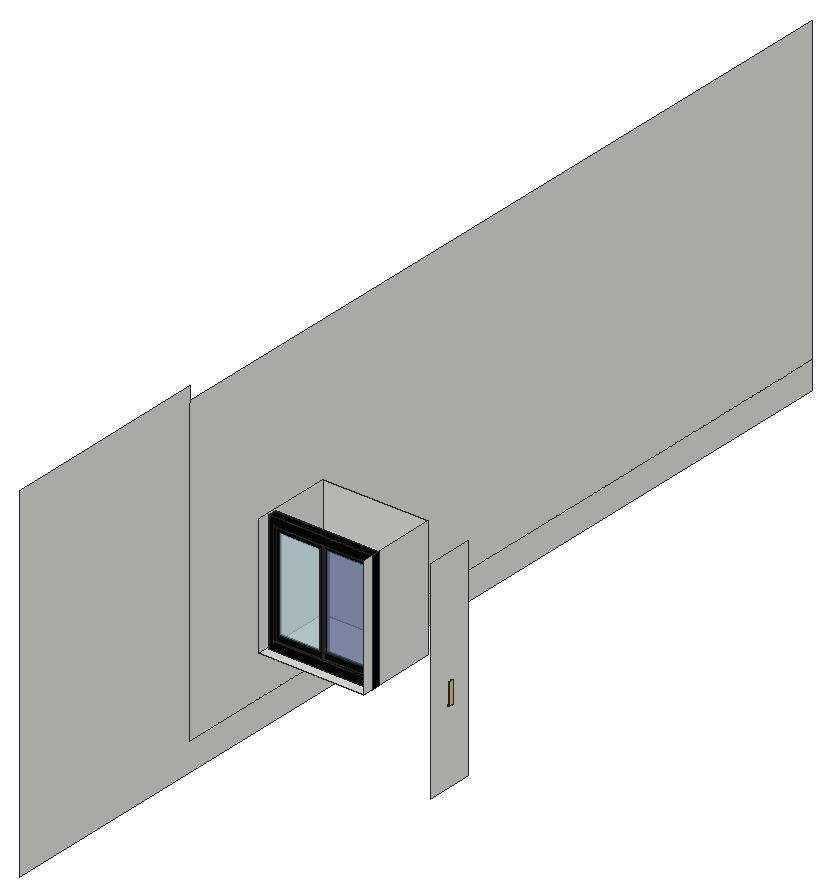
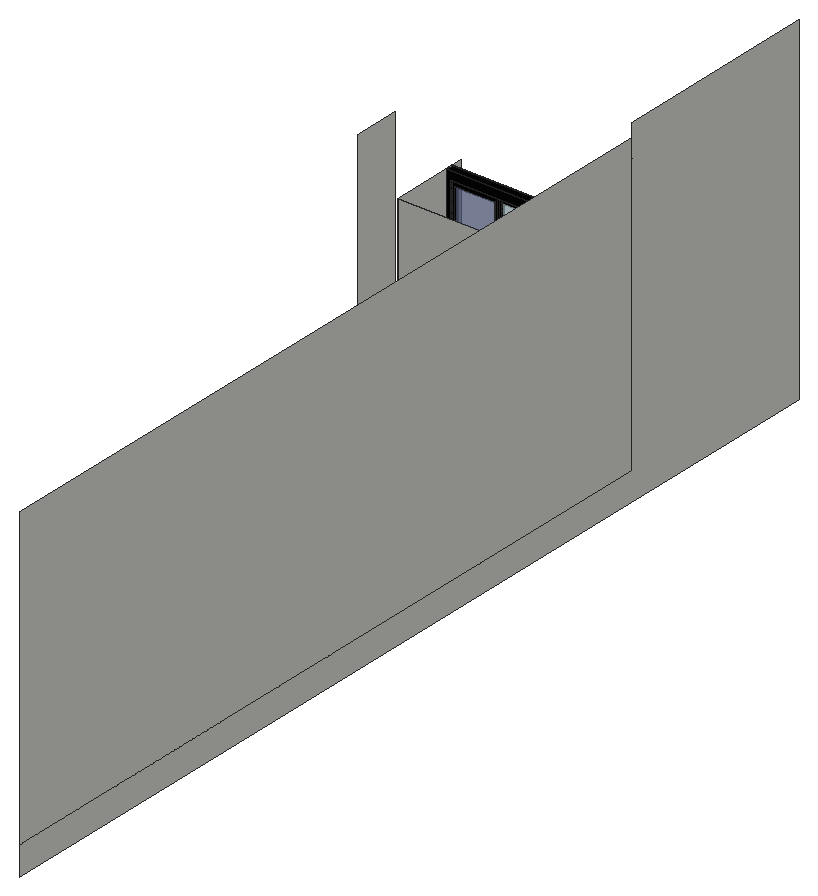
# SketchUp Ruby script. Lengths in inches.
U = 1.inch
M = Sketchup.active_model
def pt(a) = Geom::Point3d.new(a.map { |v| v * U })
def face(e, loops, mat)
  f = e.add_face(loops[0].map { |a| pt(a) })
  loops[1..].each { |l| e.add_face(l.map { |a| pt(a) }).erase! }
  f.material = f.back_material = mat if mat
  f
end
# faces: each face lists its corners as indices into pts; further lists are holes
def faces(e, pts, list, mat = nil) = list.each { |f| face(e, (f[0].is_a?(Array) ? f : [f]).map { |l| l.map { |i| pts[i] } }, mat) }
# xy, xz, yz: faces in a plane at the given z, y or x. An outline is a flat list of corners, or four numbers for a rectangle; further outlines are holes
def ring(l) = l.size == 4 ? [[l[0], l[1]], [l[2], l[1]], [l[2], l[3]], [l[0], l[3]]] : l.each_slice(2).to_a
def flat(e, list, mat, &to3) = list.each { |f| face(e, (f[0].is_a?(Array) ? f : [f]).map { |l| ring(l).map { |u, v| to3.(u, v) } }, mat) }
def xy(e, z, list, mat = nil) = flat(e, list, mat) { |x, y| [x, y, z] }
def xz(e, y, list, mat = nil) = flat(e, list, mat) { |x, z| [x, y, z] }
def yz(e, x, list, mat = nil) = flat(e, list, mat) { |y, z| [x, y, z] }
def lines(e, pts, list) = list.each { |a, b| e.add_line(pt(pts[a]), pt(pts[b])) }
# prism: a flat outline (further loops are holes) pulled along v
def prism(e, loops, v, mat = nil)
  f = face(e, loops, mat); d = Geom::Vector3d.new(v.map { |x| x * U })
  f.pushpull(f.normal.samedirection?(d) ? d.length : -d.length)
end
def box(e, o, s, mat = nil) = prism(e, [[o, [o[0] + s[0], o[1], o[2]], [o[0] + s[0], o[1] + s[1], o[2]], [o[0], o[1] + s[1], o[2]]]], [0, 0, s[2]], mat)
def at(x, y, z, deg = 0) = Geom::Transformation.translation(pt([x, y, z])) * Geom::Transformation.rotation(ORIGIN, Z_AXIS, deg.degrees)
def axes(o, x, y, z) = Geom::Transformation.new([*x, 0, *y, 0, *z, 0, *pt(o).to_a, 1])
def part(name) = M.definitions.add(name)
# library, detail: a bought-in or finely detailed component or shape, given as its bounding box
def library(name, o, s) = part(name).tap { |d| box(d.entities, o, s) }
def detail(e, o, s) = box(e.add_group.entities, o, s)
def put(e, d, t, mat = nil) = e.add_instance(d, t).tap { |i| i.material = mat if mat }
def group(e, t, mat = nil) = e.add_group.tap { |g| g.transformation = t; g.material = mat if mat }.entities
root = M.entities
M.materials.add("Generic\#5").color = [7, 6, 6]
M.materials.add("Material \#1").color = [140, 140, 140]
M.materials.add("[Translucent_Glass_Safety]").color = [204, 235, 244]
M.materials["[Translucent_Glass_Safety]"].alpha = 0.5
M.materials.add("[Translucent_Glass_Sky_Reflection]").color = [125, 138, 183]
M.materials["[Translucent_Glass_Sky_Reflection]"].alpha = 0.52
c1 = part("Sliding window")
xy(c1.entities,0,[[0,0,4.33,55.51]])
xy(c1.entities,2.76,[[0,2.76,2,27.76],[3.15,2.76,4.33,27.76],[0,27.76,0.82,52.76],[0.82,27.76,2.36,52.76],[2.36,27.76,4.33,52.76]])
xy(c1.entities,4.72,[[2,4.72,2.4,26.38],[2.76,4.72,3.15,26.38],[0.82,29.13,1.22,50.79],[1.97,29.13,2.36,50.79]])
xy(c1.entities,36.61,[[2,4.72,2.4,26.38],[2.76,4.72,3.15,26.38],[0.82,29.13,1.22,50.79],[1.97,29.13,2.36,50.79]])
xy(c1.entities,38.58,[[0,2.76,2,27.76],[3.15,2.76,4.33,27.76],[0,27.76,0.82,52.76],[0.82,27.76,2.36,52.76],[2.36,27.76,4.33,52.76]])
xy(c1.entities,41.34,[[0,0,4.33,55.51]])
xz(c1.entities,0,[[0,0,4.33,41.34]])
xz(c1.entities,2.76,[[0,2.76,2,38.58],[3.15,2.76,4.33,38.58]])
xz(c1.entities,4.72,[[2,4.72,2.4,36.61],[2.76,4.72,3.15,36.61]])
xz(c1.entities,26.38,[[2,4.72,2.4,36.61],[2.76,4.72,3.15,36.61]])
xz(c1.entities,27.76,[[0.82,2.76,2,38.58],[2,2.76,2.36,38.58],[2.36,2.76,3.15,38.58]])
xz(c1.entities,29.13,[[0.82,4.72,1.22,36.61],[1.97,4.72,2.36,36.61]])
xz(c1.entities,50.79,[[0.82,4.72,1.22,36.61],[1.97,4.72,2.36,36.61]])
xz(c1.entities,52.76,[[0,2.76,0.82,38.58],[0.82,2.76,2.36,38.58],[2.36,2.76,4.33,38.58]])
xz(c1.entities,55.51,[[0,0,4.33,41.34]])
yz(c1.entities,0,[[[0,0,55.51,41.34],[2.76,2.76,52.76,38.58]]])
yz(c1.entities,0.82,[[[27.76,2.76,52.76,38.58],[29.13,4.72,50.79,36.61]]])
yz(c1.entities,1.22,[[29.13,4.72,50.79,36.61]],"[Translucent_Glass_Sky_Reflection]")
yz(c1.entities,1.97,[[29.13,4.72,50.79,36.61]],"[Translucent_Glass_Sky_Reflection]")
yz(c1.entities,2,[[[2.76,2.76,27.76,38.58],[4.72,4.72,26.38,36.61]]])
yz(c1.entities,2.36,[[[27.76,2.76,52.76,38.58],[29.13,4.72,50.79,36.61]]])
yz(c1.entities,2.4,[[4.72,4.72,26.38,36.61]],"[Translucent_Glass_Safety]")
yz(c1.entities,2.76,[[4.72,4.72,26.38,36.61]],"[Translucent_Glass_Safety]")
yz(c1.entities,3.15,[[[2.76,2.76,27.76,38.58],[4.72,4.72,26.38,36.61]]])
yz(c1.entities,4.33,[[[0,0,55.51,41.34],[2.76,2.76,52.76,38.58]]])
c2 = library("3DGeom~4_Defintion",[-18.02,-499.97,-221.16],[36.04,1000,262.12])
c3 = part("3DGeom~5_Defintion")
xy(c3.entities,-225.24,[[-0.79,-499.98,-2.33,-499.64,7.45,-496.14],[-0.79,-499.98,7.45,-496.14,1.58,-499.88],[1.58,-499.88,7.45,-496.14,3.84,-499.16],[-2.33,-499.64,7.4,-485.75,7.45,-496.14],[3.84,-499.16,7.45,-496.14,5.85,-497.89],
  [7.45,-496.14,7.4,-485.75,8.24,-487.08],[7.45,-496.14,8.24,-487.08,8.96,-489.34],[7.45,-496.14,8.96,-489.34,9.0625,-491.71],[7.45,-496.14,9.0625,-491.71,8.55,-494.03],[-7.4,-496.08,-8.24,-494.76,2.32,-482.2],
  [-8.24,-494.76,-8.96,-492.5,2.32,-482.2],[-8.96,-492.5,-9.0625,-490.125,2.32,-482.2],[-9.0625,-490.125,-8.55,-487.81,2.32,-482.2],[-8.55,-487.81,-7.45,-485.7,2.32,-482.2],[-7.45,-485.7,-5.85,-483.95,2.32,-482.2],
  [-5.85,-483.95,-3.84,-482.68,2.32,-482.2],[-3.84,-482.68,-1.58,-481.96,2.32,-482.2],[2.32,-482.2,-1.58,-481.96,0.79,-481.86],[0,481.82,-2.35,482.13,-6.92,496.71],[0,481.82,-6.92,496.71,1.55,482.04],
  [-2.35,482.13,-4.55,483.04,-6.92,496.71],[-4.55,483.04,-6.43,484.49,-6.92,496.71],[-6.43,484.49,-7.88,486.37,-6.92,496.71],[6.92,485.12,-1.55,499.8125,7.88,495.47],[6.92,485.12,7.88,495.47,7.88,486.37],
  [-7.88,486.37,-8.79,488.57,-6.92,496.71],[7.88,486.37,7.88,495.47,8.79,488.57],[-8.79,488.57,-9.1,490.92,-6.92,496.71],[8.79,488.57,7.88,495.47,9.1,490.92],[-9.1,490.92,-8.79,493.28,-6.92,496.71],
  [9.1,490.92,7.88,495.47,8.79,493.28],[-8.79,493.28,-7.88,495.47,-6.92,496.71],[7.88,495.47,-1.55,499.8125,0,500.02],[7.88,495.47,0,500.02,2.35,499.71],[7.88,495.47,2.35,499.71,4.55,498.8],
  [7.88,495.47,4.55,498.8,6.43,497.35]],"Material \#1")
xy(c3.entities,-221.57,[[-2.33,-499.64,-5.22,-498.37,7.4,-485.75],[-5.22,-498.37,-7.4,-496.08,5.22,-483.47],[-5.22,-498.37,5.22,-483.47,7.4,-485.75],[-7.4,-496.08,2.32,-482.2,5.22,-483.47],[1.55,482.04,-6.92,496.71,-4.55,498.8],
  [1.55,482.04,-4.55,498.8,4.55,483.04],[4.55,483.04,-4.55,498.8,-1.55,499.8125],[4.55,483.04,-1.55,499.8125,6.92,485.12]],"Material \#1")
xy(c3.entities,38.05,[[-2.33,-499.64,7.4,-485.75,-5.22,-498.37],[-5.22,-498.37,5.22,-483.47,-7.4,-496.08],[-5.22,-498.37,7.4,-485.75,5.22,-483.47],[-7.4,-496.08,5.22,-483.47,2.32,-482.2],[1.55,482.04,-4.55,498.8,-6.92,496.71],
  [1.55,482.04,4.55,483.04,-4.55,498.8],[4.55,483.04,-1.55,499.8125,-4.55,498.8],[4.55,483.04,6.92,485.12,-1.55,499.8125]],"Material \#1")
xy(c3.entities,41.72,[[-0.79,-499.98,7.45,-496.14,-2.33,-499.64],[-0.79,-499.98,1.58,-499.88,7.45,-496.14],[1.58,-499.88,3.84,-499.16,7.45,-496.14],[-2.33,-499.64,7.45,-496.14,7.4,-485.75],[3.84,-499.16,5.85,-497.89,7.45,-496.14],
  [7.45,-496.14,8.24,-487.08,7.4,-485.75],[7.45,-496.14,8.55,-494.03,9.0625,-491.71],[7.45,-496.14,8.96,-489.34,8.24,-487.08],[7.45,-496.14,9.0625,-491.71,8.96,-489.34],[-7.4,-496.08,2.32,-482.2,-8.24,-494.76],
  [-8.24,-494.76,2.32,-482.2,-8.96,-492.5],[-8.96,-492.5,2.32,-482.2,-9.0625,-490.125],[-9.0625,-490.125,2.32,-482.2,-8.55,-487.81],[-8.55,-487.81,2.32,-482.2,-7.45,-485.7],[-7.45,-485.7,2.32,-482.2,-5.85,-483.95],
  [-5.85,-483.95,2.32,-482.2,-3.84,-482.68],[-3.84,-482.68,2.32,-482.2,-1.58,-481.96],[2.32,-482.2,0.79,-481.86,-1.58,-481.96],[0,481.82,-6.92,496.71,-2.35,482.13],[0,481.82,1.55,482.04,-6.92,496.71],
  [-2.35,482.13,-6.92,496.71,-4.55,483.04],[-4.55,483.04,-6.92,496.71,-6.43,484.49],[-6.43,484.49,-6.92,496.71,-7.88,486.37],[6.92,485.12,7.88,495.47,-1.55,499.8125],[6.92,485.12,7.88,486.37,7.88,495.47],
  [-7.88,486.37,-6.92,496.71,-8.79,488.57],[7.88,486.37,8.79,488.57,7.88,495.47],[-8.79,488.57,-6.92,496.71,-9.1,490.92],[8.79,488.57,9.1,490.92,7.88,495.47],[-9.1,490.92,-6.92,496.71,-8.79,493.28],
  [9.1,490.92,8.79,493.28,7.88,495.47],[-8.79,493.28,-6.92,496.71,-7.88,495.47],[7.88,495.47,0,500.02,-1.55,499.8125],[7.88,495.47,2.35,499.71,0,500.02],[7.88,495.47,4.55,498.8,2.35,499.71],
  [7.88,495.47,6.43,497.35,4.55,498.8]],"Material \#1")
xy(root,40.409,[[27.056,114.716,68.556,146.403]])
xz(root,115.852,[[100.954,47.317,100.9,47.405,100.961,47.324],[100.961,47.324,100.9,47.405,100.909,47.411],[101.228,47.368,101.214,47.403,101.237,47.374],[101.237,47.374,101.214,47.403,101.223,47.407],[101.214,47.403,101.205,47.442,101.223,47.407],
  [101.223,47.407,101.205,47.442,101.215,47.444],[101.205,47.442,101.202,47.478,101.215,47.444],[101.276,47.645,101.297,47.676,101.302,47.666]],"Material \#1")
xz(root,117.632,[[101.393,47.076,101.393,47.087,101.29,47.087],[101.29,47.087,101.291,47.098,101.193,47.118],[101.29,47.087,101.393,47.087,101.291,47.098],[101.291,47.098,101.196,47.129,101.193,47.118],[101.193,47.118,101.196,47.129,101.103,47.168],
  [101.196,47.129,101.108,47.178,101.103,47.168],[101.103,47.168,101.108,47.178,101.023,47.235],[101.108,47.178,101.03,47.244,101.023,47.235],[101.023,47.235,101.03,47.244,100.954,47.317],[101.03,47.244,100.961,47.324,100.954,47.317],
  [101.393,47.257,101.393,47.268,101.359,47.26],[101.393,47.257,101.425,47.272,101.393,47.268],[101.393,47.257,101.427,47.26,101.425,47.272],[101.359,47.26,101.36,47.272,101.326,47.271],[101.359,47.26,101.393,47.268,101.36,47.272],
  [101.326,47.271,101.33,47.282,101.297,47.288],[101.326,47.271,101.36,47.272,101.33,47.282],[101.33,47.282,101.302,47.298,101.297,47.288],[101.297,47.288,101.302,47.298,101.27,47.31],[101.302,47.298,101.276,47.319,101.27,47.31],
  [101.27,47.31,101.276,47.319,101.247,47.337],[100.954,47.317,100.961,47.324,100.9,47.405],[101.276,47.319,101.255,47.344,101.247,47.337],[100.961,47.324,100.909,47.411,100.9,47.405],[101.247,47.337,101.255,47.344,101.228,47.368],
  [101.255,47.344,101.237,47.374,101.228,47.368],[101.228,47.368,101.237,47.374,101.214,47.403],[101.237,47.374,101.223,47.407,101.214,47.403],[101.214,47.403,101.223,47.407,101.205,47.442],[100.9,47.405,100.909,47.411,100.855,47.517],
  [101.223,47.407,101.215,47.444,101.205,47.442],[100.909,47.411,100.864,47.521,100.855,47.517],[101.205,47.442,101.215,47.444,101.202,47.478],[101.215,47.444,101.212,47.478,101.202,47.478],[101.202,47.478,101.212,47.478,101.205,47.522],
  [101.212,47.478,101.215,47.52,101.205,47.522],[100.855,47.517,100.864,47.521,100.828,47.631],[101.215,47.52,101.214,47.56,101.205,47.522],[101.215,47.52,101.223,47.556,101.214,47.56],[100.864,47.521,100.838,47.633,100.828,47.631],
  [101.223,47.556,101.228,47.595,101.214,47.56],[101.223,47.556,101.237,47.59,101.228,47.595],[101.237,47.59,101.247,47.627,101.228,47.595],[101.237,47.59,101.255,47.619,101.247,47.627],[101.255,47.619,101.27,47.654,101.247,47.627],
  [101.255,47.619,101.276,47.645,101.27,47.654],[100.828,47.631,100.838,47.633,100.819,47.757],[100.838,47.633,100.828,47.758,100.819,47.757],[101.276,47.645,101.297,47.676,101.27,47.654],[101.276,47.645,101.302,47.666,101.297,47.676],
  [101.302,47.666,101.326,47.693,101.297,47.676],[101.302,47.666,101.33,47.682,101.326,47.693],[101.33,47.682,101.359,47.703,101.326,47.693],[101.33,47.682,101.36,47.692,101.359,47.703],[101.36,47.692,101.393,47.707,101.359,47.703],
  [101.36,47.692,101.393,47.695,101.393,47.707],[101.425,47.692,101.427,47.703,101.393,47.695],[101.393,47.695,101.427,47.703,101.393,47.707],[100.819,47.757,100.828,47.758,100.819,55.494],[100.828,47.758,100.828,55.493,100.819,55.494]],"Material \#1")
xz(root,146.403,[[27.056,40.409,68.556,87.784]])
yz(root,0,[[30.841,-11.1875,30.841,125.3125,114.716,125.3125,114.716,0,421.591,0,421.591,-11.1875],[114.716,0,421.591,120]])
yz(root,27.056,[[114.716,40.409,146.403,87.784]])
yz(root,68.556,[[114.716,40.409,146.403,87.784]])
yz(root,95.002,[[114.716,12.899,133.091,95.774]])
p = [[101.409,115.849,47.555],[101.409,115.873,47.555],[101.34,115.873,47.438],[101.34,115.849,47.438],[101.327,115.876,47.417],[101.327,115.851,47.417],
  [101.376,115.873,47.408],[101.376,115.849,47.408],[101.363,115.851,47.386],[101.446,115.873,47.525],[101.446,115.849,47.525],[101.3125,115.882,47.392],
  [101.3125,115.858,47.392],[101.329,115.882,47.374],[101.329,115.858,47.374],[101.349,115.882,47.362],[101.349,115.858,47.362],[101.363,115.876,47.386],
  [101.409,117.634,47.555],[101.34,117.634,47.438],[101.34,117.61,47.438],[101.409,117.61,47.555],[101.327,117.632,47.417],[101.327,117.607,47.417],
  [101.3125,117.625,47.392],[101.3125,117.601,47.392],[101.329,117.625,47.374],[101.329,117.601,47.374],[101.349,117.625,47.362],[101.349,117.601,47.362],
  [101.363,117.632,47.386],[101.363,117.607,47.386],[101.376,117.634,47.408],[101.376,117.61,47.408],[101.446,117.634,47.525],[101.446,117.61,47.525],
  [101.459,115.876,47.547],[101.459,115.851,47.547],[101.473,115.882,47.571],[101.473,115.858,47.571],[101.459,117.632,47.547],[101.459,117.607,47.547],
  [101.473,117.625,47.571],[101.473,117.601,47.571],[101.422,115.851,47.577],[101.456,115.858,47.589],[101.456,115.882,47.589],[101.437,115.882,47.601],
  [101.437,115.858,47.601],[101.422,115.876,47.577],[101.456,117.625,47.589],[101.437,117.625,47.601],[101.437,117.601,47.601],[101.456,117.601,47.589],
  [101.422,117.632,47.577],[101.422,117.607,47.577]]
faces(root,p,[[0,1,2],[2,3,0],[3,2,4],[4,5,3],[6,7,8],[7,6,9],[9,10,7],[5,4,11],
  [11,12,5],[12,11,13],[13,14,12],[14,13,15],[15,16,14],[16,15,17],[17,8,16],[8,17,6],
  [18,19,20],[20,21,18],[19,22,23],[23,20,19],[22,24,25],[25,23,22],[24,26,27],[27,25,24],
  [26,28,29],[29,27,26],[28,30,31],[31,29,28],[30,32,33],[33,31,30],[32,34,35],[35,33,32],
  [10,9,36],[36,37,10],[37,36,38],[38,39,37],[34,40,41],[41,35,34],[40,42,43],[43,41,40],
  [1,0,44],[45,46,47],[47,48,45],[48,47,49],[49,44,48],[44,49,1],[39,38,46],[46,45,39],
  [50,51,52],[52,53,50],[51,54,55],[55,52,51],[54,18,21],[21,55,54],[42,50,53],[53,43,42]],"Material \#1")
put(root,c1,axes([27.87,122.1,40.41],[0,-0.7372,0],[0.7372,0,0],[0,0,1.14602]),"Generic\#5")
put(root,c2,axes([101.39,117.36,51.625],[0.00728,0,0],[0,0,0.0086],[0,0.00681,0]),"Material \#1")
put(root,c3,axes([101.39,117.36,51.625],[0.00715,0,0],[0,0,0.00844],[0,0.00669,0]),"Material \#1")
